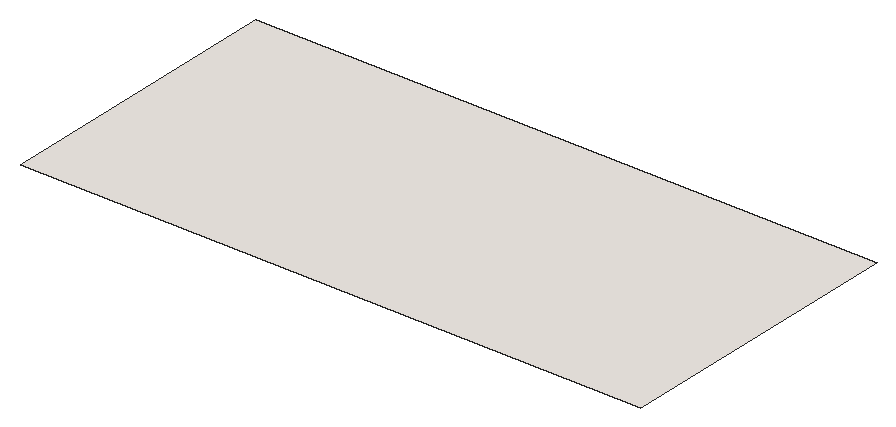
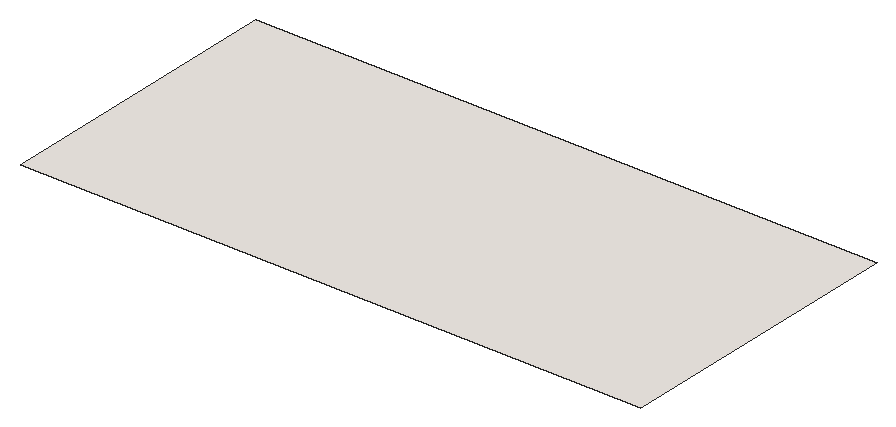
# SketchUp Ruby script. Lengths in inches.
U = 1.inch
M = Sketchup.active_model
def pt(a) = Geom::Point3d.new(a.map { |v| v * U })
def face(e, loops, mat)
  f = e.add_face(loops[0].map { |a| pt(a) })
  loops[1..].each { |l| e.add_face(l.map { |a| pt(a) }).erase! }
  f.material = f.back_material = mat if mat
  f
end
# faces: each face lists its corners as indices into pts; further lists are holes
def faces(e, pts, list, mat = nil) = list.each { |f| face(e, (f[0].is_a?(Array) ? f : [f]).map { |l| l.map { |i| pts[i] } }, mat) }
# xy, xz, yz: faces in a plane at the given z, y or x. An outline is a flat list of corners, or four numbers for a rectangle; further outlines are holes
def ring(l) = l.size == 4 ? [[l[0], l[1]], [l[2], l[1]], [l[2], l[3]], [l[0], l[3]]] : l.each_slice(2).to_a
def flat(e, list, mat, &to3) = list.each { |f| face(e, (f[0].is_a?(Array) ? f : [f]).map { |l| ring(l).map { |u, v| to3.(u, v) } }, mat) }
def xy(e, z, list, mat = nil) = flat(e, list, mat) { |x, y| [x, y, z] }
def xz(e, y, list, mat = nil) = flat(e, list, mat) { |x, z| [x, y, z] }
def yz(e, x, list, mat = nil) = flat(e, list, mat) { |y, z| [x, y, z] }
def lines(e, pts, list) = list.each { |a, b| e.add_line(pt(pts[a]), pt(pts[b])) }
# prism: a flat outline (further loops are holes) pulled along v
def prism(e, loops, v, mat = nil)
  f = face(e, loops, mat); d = Geom::Vector3d.new(v.map { |x| x * U })
  f.pushpull(f.normal.samedirection?(d) ? d.length : -d.length)
end
def box(e, o, s, mat = nil) = prism(e, [[o, [o[0] + s[0], o[1], o[2]], [o[0] + s[0], o[1] + s[1], o[2]], [o[0], o[1] + s[1], o[2]]]], [0, 0, s[2]], mat)
def at(x, y, z, deg = 0) = Geom::Transformation.translation(pt([x, y, z])) * Geom::Transformation.rotation(ORIGIN, Z_AXIS, deg.degrees)
def axes(o, x, y, z) = Geom::Transformation.new([*x, 0, *y, 0, *z, 0, *pt(o).to_a, 1])
def part(name) = M.definitions.add(name)
# library, detail: a bought-in or finely detailed component or shape, given as its bounding box
def library(name, o, s) = part(name).tap { |d| box(d.entities, o, s) }
def detail(e, o, s) = box(e.add_group.entities, o, s)
def put(e, d, t, mat = nil) = e.add_instance(d, t).tap { |i| i.material = mat if mat }
def group(e, t, mat = nil) = e.add_group.tap { |g| g.transformation = t; g.material = mat if mat }.entities
root = M.entities
M.materials.add("0001 AP 9436 AIR BREEZE").color = [243, 237, 232]
xy(root,108,[[23.91,40.5,23.83,40.51,23.75,40.51,23.51,40.54,23.4375,40.55,23.36,40.57,23.28,40.59,23.21,40.61,23.13,40.63,23.06,40.65,22.98,40.68,22.91,40.71,22.84,40.73,22.76,40.77,22.69,40.8,22.625,40.83,22.55,40.87,22.49,40.91,22.35,40.99,22.29,41.04,22.22,41.08,21.98,41.28,21.87,41.39,21.8125,41.45,21.76,41.5,21.61,41.6875,21.5625,41.75,21.52,41.8125,21.48,41.88,21.43,41.95,21.39,42.01,21.36,42.08,21.32,42.15,21.29,42.22,21.25,42.29,21.22,42.37,21.19,42.44,21.17,42.51,21.14,42.59,21.12,42.66,21.0625,42.89,21.05,42.97,21.03,43.05,21.01,43.2,21.01,43.28,21,43.36,21,43.59,21.01,43.67,21.01,43.75,21.04,43.99,21.05,44.0625,21.07,44.14,21.09,44.22,21.11,44.29,21.13,44.37,21.15,44.44,21.18,44.52,21.21,44.59,21.23,44.66,21.27,44.74,21.3,44.81,21.33,44.875,21.37,44.95,21.41,45.01,21.49,45.15,21.54,45.21,21.58,45.28,21.78,45.52,21.89,45.63,21.95,45.6875,22,45.74,22.1875,45.89,22.25,45.9375,22.3125,45.98,22.38,46.02,22.45,46.07,22.51,46.11,22.58,46.14,22.65,46.18,22.72,46.21,22.79,46.25,22.87,46.28,22.94,46.31,23.01,46.33,23.09,46.36,23.16,46.38,23.39,46.4375,23.47,46.45,23.55,46.47,23.7,46.49,23.78,46.49,23.86,46.5,24.09,46.5,24.17,46.49,24.25,46.49,24.49,46.46,24.5625,46.45,24.64,46.43,24.72,46.41,24.79,46.39,24.87,46.37,24.94,46.35,25.02,46.32,25.09,46.29,25.16,46.27,25.24,46.23,25.31,46.2,25.375,46.17,25.45,46.13,25.51,46.09,25.65,46.01,25.71,45.96,25.78,45.92,26.02,45.72,26.13,45.61,26.1875,45.55,26.24,45.5,26.39,45.3125,26.4375,45.25,26.48,45.1875,26.52,45.12,26.57,45.05,26.61,44.99,26.64,44.92,26.68,44.85,26.71,44.78,26.75,44.71,26.78,44.63,26.81,44.56,26.83,44.49,26.86,44.41,26.88,44.34,26.9375,44.11,26.95,44.03,26.97,43.95,26.99,43.8,26.99,43.72,27,43.64,27,43.41,26.99,43.33,26.99,43.25,26.96,43.01,26.95,42.9375,26.93,42.86,26.91,42.78,26.89,42.71,26.87,42.63,26.85,42.56,26.82,42.48,26.79,42.41,26.77,42.34,26.73,42.26,26.7,42.19,26.67,42.125,26.63,42.05,26.59,41.99,26.51,41.85,26.46,41.79,26.42,41.72,26.22,41.48,26.11,41.37,26.05,41.3125,26,41.26,25.8125,41.11,25.75,41.0625,25.6875,41.02,25.62,40.98,25.55,40.93,25.49,40.89,25.42,40.86,25.35,40.82,25.28,40.79,25.21,40.75,25.13,40.72,25.06,40.69,24.99,40.67,24.91,40.64,24.84,40.62,24.61,40.5625,24.53,40.55,24.45,40.53,24.3,40.51,24.22,40.51,24.14,40.5],[68.91,40.5,68.83,40.51,68.75,40.51,68.51,40.54,68.4375,40.55,68.36,40.57,68.28,40.59,68.21,40.61,68.13,40.63,68.06,40.65,67.98,40.68,67.91,40.71,67.84,40.73,67.76,40.77,67.69,40.8,67.625,40.83,67.55,40.87,67.49,40.91,67.35,40.99,67.29,41.04,67.22,41.08,66.98,41.28,66.87,41.39,66.8125,41.45,66.76,41.5,66.61,41.6875,66.5625,41.75,66.52,41.8125,66.48,41.88,66.43,41.95,66.39,42.01,66.36,42.08,66.32,42.15,66.29,42.22,66.25,42.29,66.22,42.37,66.19,42.44,66.17,42.51,66.14,42.59,66.12,42.66,66.0625,42.89,66.05,42.97,66.03,43.05,66.01,43.2,66.01,43.28,66,43.36,66,43.59,66.01,43.67,66.01,43.75,66.04,43.99,66.05,44.0625,66.07,44.14,66.09,44.22,66.11,44.29,66.13,44.37,66.15,44.44,66.18,44.52,66.21,44.59,66.23,44.66,66.27,44.74,66.3,44.81,66.33,44.875,66.37,44.95,66.41,45.01,66.49,45.15,66.54,45.21,66.58,45.28,66.78,45.52,66.89,45.63,66.95,45.6875,67,45.74,67.1875,45.89,67.25,45.9375,67.3125,45.98,67.38,46.02,67.45,46.07,67.51,46.11,67.58,46.14,67.65,46.18,67.72,46.21,67.79,46.25,67.87,46.28,67.94,46.31,68.01,46.33,68.09,46.36,68.16,46.38,68.39,46.4375,68.47,46.45,68.55,46.47,68.7,46.49,68.78,46.49,68.86,46.5,69.09,46.5,69.17,46.49,69.25,46.49,69.49,46.46,69.5625,46.45,69.64,46.43,69.72,46.41,69.79,46.39,69.87,46.37,69.94,46.35,70.02,46.32,70.09,46.29,70.16,46.27,70.24,46.23,70.31,46.2,70.375,46.17,70.45,46.13,70.51,46.09,70.65,46.01,70.71,45.96,70.78,45.92,71.02,45.72,71.13,45.61,71.1875,45.55,71.24,45.5,71.39,45.3125,71.4375,45.25,71.48,45.1875,71.52,45.12,71.57,45.05,71.61,44.99,71.64,44.92,71.68,44.85,71.71,44.78,71.75,44.71,71.78,44.63,71.81,44.56,71.83,44.49,71.86,44.41,71.88,44.34,71.9375,44.11,71.95,44.03,71.97,43.95,71.99,43.8,71.99,43.72,72,43.64,72,43.41,71.99,43.33,71.99,43.25,71.96,43.01,71.95,42.9375,71.93,42.86,71.91,42.78,71.89,42.71,71.87,42.63,71.85,42.56,71.82,42.48,71.79,42.41,71.77,42.34,71.73,42.26,71.7,42.19,71.67,42.125,71.63,42.05,71.59,41.99,71.51,41.85,71.46,41.79,71.42,41.72,71.22,41.48,71.11,41.37,71.05,41.3125,71,41.26,70.8125,41.11,70.75,41.0625,70.6875,41.02,70.62,40.98,70.55,40.93,70.49,40.89,70.42,40.86,70.35,40.82,70.28,40.79,70.21,40.75,70.13,40.72,70.06,40.69,69.99,40.67,69.91,40.64,69.84,40.62,69.61,40.5625,69.53,40.55,69.45,40.53,69.3,40.51,69.22,40.51,69.14,40.5],[113.91,40.5,113.83,40.51,113.75,40.51,113.51,40.54,113.4375,40.55,113.36,40.57,113.28,40.59,113.21,40.61,113.13,40.63,113.06,40.65,112.98,40.68,112.91,40.71,112.84,40.73,112.76,40.77,112.69,40.8,112.625,40.83,112.55,40.87,112.49,40.91,112.35,40.99,112.29,41.04,112.22,41.08,111.98,41.28,111.87,41.39,111.8125,41.45,111.76,41.5,111.61,41.6875,111.5625,41.75,111.52,41.8125,111.48,41.88,111.43,41.95,111.39,42.01,111.36,42.08,111.32,42.15,111.29,42.22,111.25,42.29,111.22,42.37,111.19,42.44,111.17,42.51,111.14,42.59,111.12,42.66,111.0625,42.89,111.05,42.97,111.03,43.05,111.01,43.2,111.01,43.28,111,43.36,111,43.59,111.01,43.67,111.01,43.75,111.04,43.99,111.05,44.0625,111.07,44.14,111.09,44.22,111.11,44.29,111.13,44.37,111.15,44.44,111.18,44.52,111.21,44.59,111.23,44.66,111.27,44.74,111.3,44.81,111.33,44.875,111.37,44.95,111.41,45.01,111.49,45.15,111.54,45.21,111.58,45.28,111.78,45.52,111.89,45.63,111.95,45.6875,112,45.74,112.1875,45.89,112.25,45.9375,112.3125,45.98,112.38,46.02,112.45,46.07,112.51,46.11,112.58,46.14,112.65,46.18,112.72,46.21,112.79,46.25,112.87,46.28,112.94,46.31,113.01,46.33,113.09,46.36,113.16,46.38,113.39,46.4375,113.47,46.45,113.55,46.47,113.7,46.49,113.78,46.49,113.86,46.5,114.09,46.5,114.17,46.49,114.25,46.49,114.49,46.46,114.5625,46.45,114.64,46.43,114.72,46.41,114.79,46.39,114.87,46.37,114.94,46.35,115.02,46.32,115.09,46.29,115.16,46.27,115.24,46.23,115.31,46.2,115.375,46.17,115.45,46.13,115.51,46.09,115.65,46.01,115.71,45.96,115.78,45.92,116.02,45.72,116.13,45.61,116.1875,45.55,116.24,45.5,116.39,45.3125,116.4375,45.25,116.48,45.1875,116.52,45.12,116.57,45.05,116.61,44.99,116.64,44.92,116.68,44.85,116.71,44.78,116.75,44.71,116.78,44.63,116.81,44.56,116.83,44.49,116.86,44.41,116.88,44.34,116.9375,44.11,116.95,44.03,116.97,43.95,116.99,43.8,116.99,43.72,117,43.64,117,43.41,116.99,43.33,116.99,43.25,116.96,43.01,116.95,42.9375,116.93,42.86,116.91,42.78,116.89,42.71,116.87,42.63,116.85,42.56,116.82,42.48,116.79,42.41,116.77,42.34,116.73,42.26,116.7,42.19,116.67,42.125,116.63,42.05,116.59,41.99,116.51,41.85,116.46,41.79,116.42,41.72,116.22,41.48,116.11,41.37,116.05,41.3125,116,41.26,115.8125,41.11,115.75,41.0625,115.6875,41.02,115.62,40.98,115.55,40.93,115.49,40.89,115.42,40.86,115.35,40.82,115.28,40.79,115.21,40.75,115.13,40.72,115.06,40.69,114.99,40.67,114.91,40.64,114.84,40.62,114.61,40.5625,114.53,40.55,114.45,40.53,114.3,40.51,114.22,40.51,114.14,40.5]],"0001 AP 9436 AIR BREEZE")
xy(root,112,[[0,0,183,87]],"0001 AP 9436 AIR BREEZE")
xz(root,40.5,[[113.91,106,113.98,108],[113.98,106,114.0625,108],[114.0625,106,114.14,108]],"0001 AP 9436 AIR BREEZE")
xz(root,40.51,[[113.75,106,113.83,108],[114.22,106,114.3,108]],"0001 AP 9436 AIR BREEZE")
xz(root,46.49,[[113.7,106,113.78,108],[114.17,106,114.25,108]],"0001 AP 9436 AIR BREEZE")
xz(root,46.5,[[113.86,106,113.9375,108],[113.9375,106,114.02,108],[114.02,106,114.09,108]],"0001 AP 9436 AIR BREEZE")
yz(root,111,[[43.36,106,43.4375,108],[43.4375,106,43.52,108],[43.52,106,43.59,108]],"0001 AP 9436 AIR BREEZE")
yz(root,111.01,[[43.2,106,43.28,108],[43.67,106,43.75,108]],"0001 AP 9436 AIR BREEZE")
p = [[113.51,40.54,106],[113.4375,40.55,106],[113.4375,40.55,108],[113.51,40.54,108],[113.59,40.53,106],[113.59,40.53,108],
  [113.67,40.52,106],[113.67,40.52,108],[113.75,40.51,106],[113.75,40.51,108],[113.91,40.5,106],[113.83,40.51,106],
  [113.83,40.51,108],[113.91,40.5,108],[114.22,40.51,106],[114.14,40.5,106],[114.14,40.5,108],[114.22,40.51,108],
  [114.375,40.52,106],[114.3,40.51,106],[114.3,40.51,108],[114.375,40.52,108],[114.45,40.53,106],[114.45,40.53,108],
  [114.53,40.55,106],[114.53,40.55,108],[114.61,40.5625,106],[114.61,40.5625,108],[113.13,40.63,106],[113.06,40.65,106],
  [113.06,40.65,108],[113.13,40.63,108],[113.21,40.61,106],[113.21,40.61,108],[113.28,40.59,106],[113.28,40.59,108],
  [113.36,40.57,106],[113.36,40.57,108],[114.68,40.58,106],[114.68,40.58,108],[114.76,40.6,106],[114.76,40.6,108],
  [114.84,40.62,106],[114.84,40.62,108],[114.91,40.64,106],[114.91,40.64,108],[114.99,40.67,106],[114.99,40.67,108],
  [112.84,40.73,106],[112.76,40.77,106],[112.76,40.77,108],[112.84,40.73,108],[112.91,40.71,106],[112.91,40.71,108],
  [112.98,40.68,106],[112.98,40.68,108],[115.06,40.69,106],[115.06,40.69,108],[115.13,40.72,106],[115.13,40.72,108],
  [115.21,40.75,106],[115.21,40.75,108],[112.625,40.83,106],[112.55,40.87,106],[112.55,40.87,108],[112.625,40.83,108],
  [112.69,40.8,106],[112.69,40.8,108],[115.28,40.79,106],[115.28,40.79,108],[115.35,40.82,106],[115.35,40.82,108],
  [115.42,40.86,106],[115.42,40.86,108],[112.49,40.91,106],[112.42,40.95,106],[112.42,40.95,108],[112.49,40.91,108],
  [115.49,40.89,106],[115.49,40.89,108],[115.55,40.93,106],[115.55,40.93,108],[115.62,40.98,106],[115.62,40.98,108],
  [112.29,41.04,106],[112.22,41.08,106],[112.22,41.08,108],[112.29,41.04,108],[112.35,40.99,106],[112.35,40.99,108],
  [115.6875,41.02,106],[115.6875,41.02,108],[115.75,41.0625,106],[115.75,41.0625,108],[112.16,41.13,106],[112.1,41.18,106],
  [112.1,41.18,108],[112.16,41.13,108],[115.8125,41.11,106],[115.8125,41.11,108],[115.875,41.16,106],[115.875,41.16,108],
  [112.04,41.23,106],[111.98,41.28,106],[111.98,41.28,108],[112.04,41.23,108],[115.9375,41.21,106],[115.9375,41.21,108],
  [116,41.26,106],[116,41.26,108],[111.92,41.34,106],[111.87,41.39,106],[111.87,41.39,108],[111.92,41.34,108],
  [116.05,41.3125,106],[116.05,41.3125,108],[116.11,41.37,106],[116.11,41.37,108],[111.8125,41.45,106],[111.76,41.5,106],
  [111.76,41.5,108],[111.8125,41.45,108],[116.16,41.42,106],[116.16,41.42,108],[116.22,41.48,106],[116.22,41.48,108],
  [111.71,41.5625,106],[111.71,41.5625,108],[116.27,41.54,106],[116.27,41.54,108],[116.32,41.6,106],[116.32,41.6,108],
  [111.66,41.625,106],[111.61,41.6875,106],[111.61,41.6875,108],[111.66,41.625,108],[116.37,41.66,106],[116.37,41.66,108],
  [111.5625,41.75,106],[111.52,41.8125,106],[111.52,41.8125,108],[111.5625,41.75,108],[116.42,41.72,106],[116.42,41.72,108],
  [116.46,41.79,106],[116.46,41.79,108],[111.48,41.88,106],[111.48,41.88,108],[116.51,41.85,106],[116.51,41.85,108],
  [111.43,41.95,106],[111.39,42.01,106],[111.39,42.01,108],[111.43,41.95,108],[116.55,41.92,106],[116.55,41.92,108],
  [116.59,41.99,106],[116.59,41.99,108],[111.36,42.08,106],[111.36,42.08,108],[116.63,42.05,106],[116.63,42.05,108],
  [111.32,42.15,106],[111.32,42.15,108],[116.67,42.125,106],[116.67,42.125,108],[116.7,42.19,106],[116.7,42.19,108],
  [111.29,42.22,106],[111.25,42.29,106],[111.25,42.29,108],[111.29,42.22,108],[116.73,42.26,106],[116.73,42.26,108],
  [111.22,42.37,106],[111.22,42.37,108],[116.77,42.34,106],[116.77,42.34,108],[116.79,42.41,106],[116.79,42.41,108],
  [111.19,42.44,106],[111.17,42.51,106],[111.17,42.51,108],[111.19,42.44,108],[116.82,42.48,106],[116.82,42.48,108],
  [111.14,42.59,106],[111.14,42.59,108],[116.85,42.56,106],[116.85,42.56,108],[111.12,42.66,106],[111.12,42.66,108],
  [116.87,42.63,106],[116.87,42.63,108],[116.89,42.71,106],[116.89,42.71,108],[111.1,42.74,106],[111.08,42.82,106],
  [111.08,42.82,108],[111.1,42.74,108],[116.91,42.78,106],[116.91,42.78,108],[111.0625,42.89,106],[111.0625,42.89,108],
  [116.93,42.86,106],[116.93,42.86,108],[111.05,42.97,106],[111.05,42.97,108],[116.95,42.9375,106],[116.95,42.9375,108],
  [116.96,43.01,106],[116.96,43.01,108],[111.03,43.05,106],[111.02,43.125,106],[111.02,43.125,108],[111.03,43.05,108],
  [116.97,43.09,106],[116.97,43.09,108],[111.01,43.2,106],[111.01,43.2,108],[116.98,43.17,106],[116.98,43.17,108],
  [116.99,43.25,106],[116.99,43.25,108],[111.01,43.28,106],[111,43.36,106],[111,43.36,108],[111.01,43.28,108],
  [111,43.59,106],[111.01,43.67,106],[111.01,43.67,108],[111,43.59,108],[111.01,43.75,106],[111.02,43.83,106],
  [111.02,43.83,108],[111.01,43.75,108],[111.03,43.91,106],[111.03,43.91,108],[116.98,43.875,106],[116.99,43.8,106],
  [116.99,43.8,108],[116.98,43.875,108],[111.04,43.99,106],[111.04,43.99,108],[116.97,43.95,106],[116.97,43.95,108],
  [111.05,44.0625,106],[111.05,44.0625,108],[116.9375,44.11,106],[116.95,44.03,106],[116.95,44.03,108],[116.9375,44.11,108],
  [111.07,44.14,106],[111.07,44.14,108],[111.09,44.22,106],[111.09,44.22,108],[116.92,44.18,106],[116.92,44.18,108],
  [111.11,44.29,106],[111.11,44.29,108],[116.9,44.26,106],[116.9,44.26,108],[111.13,44.37,106],[111.13,44.37,108],
  [116.86,44.41,106],[116.88,44.34,106],[116.88,44.34,108],[116.86,44.41,108],[111.15,44.44,106],[111.15,44.44,108],
  [111.18,44.52,106],[111.18,44.52,108],[116.83,44.49,106],[116.83,44.49,108],[111.21,44.59,106],[111.21,44.59,108],
  [116.81,44.56,106],[116.81,44.56,108],[111.23,44.66,106],[111.23,44.66,108],[116.75,44.71,106],[116.78,44.63,106],
  [116.78,44.63,108],[116.75,44.71,108],[111.27,44.74,106],[111.27,44.74,108],[111.3,44.81,106],[111.3,44.81,108],
  [116.71,44.78,106],[116.71,44.78,108],[111.33,44.875,106],[111.33,44.875,108],[116.64,44.92,106],[116.68,44.85,106],
  [116.68,44.85,108],[116.64,44.92,108],[111.37,44.95,106],[111.37,44.95,108],[111.41,45.01,106],[111.41,45.01,108],
  [116.61,44.99,106],[116.61,44.99,108],[111.45,45.08,106],[111.45,45.08,108],[116.57,45.05,106],[116.57,45.05,108],
  [111.49,45.15,106],[111.49,45.15,108],[111.54,45.21,106],[111.54,45.21,108],[116.48,45.1875,106],[116.52,45.12,106],
  [116.52,45.12,108],[116.48,45.1875,108],[111.58,45.28,106],[111.58,45.28,108],[116.4375,45.25,106],[116.4375,45.25,108],
  [111.63,45.34,106],[111.63,45.34,108],[111.68,45.4,106],[111.68,45.4,108],[116.34,45.375,106],[116.39,45.3125,106],
  [116.39,45.3125,108],[116.34,45.375,108],[111.73,45.46,106],[111.73,45.46,108],[116.24,45.5,106],[116.29,45.4375,106],
  [116.29,45.4375,108],[116.24,45.5,108],[111.78,45.52,106],[111.78,45.52,108],[111.84,45.58,106],[111.84,45.58,108],
  [116.1875,45.55,106],[116.1875,45.55,108],[111.89,45.63,106],[111.89,45.63,108],[111.95,45.6875,106],[111.95,45.6875,108],
  [116.08,45.66,106],[116.13,45.61,106],[116.13,45.61,108],[116.08,45.66,108],[112,45.74,106],[112,45.74,108],
  [112.0625,45.79,106],[112.0625,45.79,108],[115.96,45.77,106],[116.02,45.72,106],[116.02,45.72,108],[115.96,45.77,108],
  [112.125,45.84,106],[112.125,45.84,108],[112.1875,45.89,106],[112.1875,45.89,108],[115.84,45.87,106],[115.9,45.82,106],
  [115.9,45.82,108],[115.84,45.87,108],[70.71,45.96,106],[70.78,45.92,106],[70.78,45.92,108],[70.71,45.96,108],
  [112.25,45.9375,106],[112.25,45.9375,108],[112.3125,45.98,106],[112.3125,45.98,108],[115.71,45.96,106],[115.78,45.92,106],
  [115.78,45.92,108],[115.71,45.96,108],[70.51,46.09,106],[70.58,46.05,106],[70.58,46.05,108],[70.51,46.09,108],
  [70.65,46.01,106],[70.65,46.01,108],[112.38,46.02,106],[112.38,46.02,108],[112.45,46.07,106],[112.45,46.07,108],
  [115.51,46.09,106],[115.58,46.05,106],[115.58,46.05,108],[115.51,46.09,108],[115.65,46.01,106],[115.65,46.01,108],
  [70.375,46.17,106],[70.45,46.13,106],[70.45,46.13,108],[70.375,46.17,108],[112.51,46.11,106],[112.51,46.11,108],
  [112.58,46.14,106],[112.58,46.14,108],[112.65,46.18,106],[112.65,46.18,108],[115.375,46.17,106],[115.45,46.13,106],
  [115.45,46.13,108],[115.375,46.17,108],[70.16,46.27,106],[70.24,46.23,106],[70.24,46.23,108],[70.16,46.27,108],
  [70.31,46.2,106],[70.31,46.2,108],[112.72,46.21,106],[112.72,46.21,108],[112.79,46.25,106],[112.79,46.25,108],
  [112.87,46.28,106],[112.87,46.28,108],[115.16,46.27,106],[115.24,46.23,106],[115.24,46.23,108],[115.16,46.27,108],
  [115.31,46.2,106],[115.31,46.2,108],[70.02,46.32,106],[70.09,46.29,106],[70.09,46.29,108],[70.02,46.32,108],
  [112.94,46.31,106],[112.94,46.31,108],[113.01,46.33,106],[113.01,46.33,108],[113.09,46.36,106],[113.09,46.36,108],
  [114.87,46.37,106],[114.94,46.35,106],[114.94,46.35,108],[114.87,46.37,108],[115.02,46.32,106],[115.02,46.32,108],
  [115.09,46.29,106],[115.09,46.29,108],[113.16,46.38,106],[113.16,46.38,108],[113.24,46.4,106],[113.24,46.4,108],
  [113.32,46.42,106],[113.32,46.42,108],[113.39,46.4375,106],[113.39,46.4375,108],[113.47,46.45,106],[113.47,46.45,108],
  [114.49,46.46,106],[114.5625,46.45,106],[114.5625,46.45,108],[114.49,46.46,108],[114.64,46.43,106],[114.64,46.43,108],
  [114.72,46.41,106],[114.72,46.41,108],[114.79,46.39,106],[114.79,46.39,108],[113.55,46.47,106],[113.55,46.47,108],
  [113.625,46.48,106],[113.625,46.48,108],[113.7,46.49,106],[113.7,46.49,108],[113.78,46.49,106],[113.86,46.5,106],
  [113.86,46.5,108],[113.78,46.49,108],[114.09,46.5,106],[114.17,46.49,106],[114.17,46.49,108],[114.09,46.5,108],
  [114.25,46.49,106],[114.33,46.48,106],[114.33,46.48,108],[114.25,46.49,108],[114.41,46.47,106],[114.41,46.47,108]]
faces(root,p,[[0,1,2,3],[4,0,3,5],[6,4,5,7],[8,6,7,9],[10,11,12,13],[14,15,16,17],[18,19,20,21],[22,18,21,23],
  [24,22,23,25],[26,24,25,27],[28,29,30,31],[32,28,31,33],[34,32,33,35],[36,34,35,37],[1,36,37,2],[38,26,27,39],
  [40,38,39,41],[42,40,41,43],[44,42,43,45],[46,44,45,47],[48,49,50,51],[52,48,51,53],[54,52,53,55],[29,54,55,30],
  [56,46,47,57],[58,56,57,59],[60,58,59,61],[62,63,64,65],[66,62,65,67],[49,66,67,50],[68,60,61,69],[70,68,69,71],
  [72,70,71,73],[74,75,76,77],[63,74,77,64],[78,72,73,79],[80,78,79,81],[82,80,81,83],[84,85,86,87],[88,84,87,89],
  [75,88,89,76],[90,82,83,91],[92,90,91,93],[94,95,96,97],[85,94,97,86],[98,92,93,99],[100,98,99,101],[102,103,104,105],
  [95,102,105,96],[106,100,101,107],[108,106,107,109],[110,111,112,113],[103,110,113,104],[114,108,109,115],[116,114,115,117],[118,119,120,121],
  [111,118,121,112],[122,116,117,123],[124,122,123,125],[119,126,127,120],[128,124,125,129],[130,128,129,131],[132,133,134,135],[126,132,135,127],
  [136,130,131,137],[138,139,140,141],[133,138,141,134],[142,136,137,143],[144,142,143,145],[139,146,147,140],[148,144,145,149],[150,151,152,153],
  [146,150,153,147],[154,148,149,155],[156,154,155,157],[151,158,159,152],[160,156,157,161],[158,162,163,159],[164,160,161,165],[166,164,165,167],
  [168,169,170,171],[162,168,171,163],[172,166,167,173],[169,174,175,170],[176,172,173,177],[178,176,177,179],[180,181,182,183],[174,180,183,175],
  [184,178,179,185],[181,186,187,182],[188,184,185,189],[186,190,191,187],[192,188,189,193],[194,192,193,195],[196,197,198,199],[190,196,199,191],
  [200,194,195,201],[197,202,203,198],[204,200,201,205],[202,206,207,203],[208,204,205,209],[210,208,209,211],[212,213,214,215],[206,212,215,207],
  [216,210,211,217],[213,218,219,214],[220,216,217,221],[222,220,221,223],[224,225,226,227],[228,229,230,231],[232,233,234,235],[233,236,237,234],
  [238,239,240,241],[236,242,243,237],[244,238,241,245],[242,246,247,243],[248,249,250,251],[249,244,245,250],[246,252,253,247],[252,254,255,253],
  [256,248,251,257],[254,258,259,255],[260,256,257,261],[258,262,263,259],[264,265,266,267],[265,260,261,266],[262,268,269,263],[268,270,271,269],
  [272,264,267,273],[270,274,275,271],[276,272,273,277],[274,278,279,275],[280,281,282,283],[281,276,277,282],[278,284,285,279],[284,286,287,285],
  [288,280,283,289],[286,290,291,287],[292,293,294,295],[293,288,289,294],[290,296,297,291],[296,298,299,297],[300,292,295,301],[298,302,303,299],
  [304,300,301,305],[302,306,307,303],[306,308,309,307],[310,311,312,313],[311,304,305,312],[308,314,315,309],[316,310,313,317],[314,318,319,315],
  [318,320,321,319],[322,323,324,325],[323,316,317,324],[320,326,327,321],[328,329,330,331],[329,322,325,330],[326,332,333,327],[332,334,335,333],
  [336,328,331,337],[334,338,339,335],[338,340,341,339],[342,343,344,345],[343,336,337,344],[340,346,347,341],[346,348,349,347],[350,351,352,353],
  [351,342,345,352],[348,354,355,349],[354,356,357,355],[358,359,360,361],[359,350,353,360],[362,363,364,365],[356,366,367,357],[366,368,369,367],
  [370,371,372,373],[371,358,361,372],[374,375,376,377],[375,378,379,376],[378,362,365,379],[368,380,381,369],[380,382,383,381],[384,385,386,387],
  [385,388,389,386],[388,370,373,389],[390,391,392,393],[391,374,377,392],[382,394,395,383],[394,396,397,395],[396,398,399,397],[400,401,402,403],
  [401,384,387,402],[404,405,406,407],[405,408,409,406],[408,390,393,409],[398,410,411,399],[410,412,413,411],[412,414,415,413],[416,417,418,419],
  [417,420,421,418],[420,400,403,421],[422,423,424,425],[423,404,407,424],[414,426,427,415],[426,428,429,427],[428,430,431,429],[432,433,434,435],
  [433,436,437,434],[436,438,439,437],[438,416,419,439],[430,440,441,431],[440,442,443,441],[442,444,445,443],[444,446,447,445],[446,448,449,447],
  [450,451,452,453],[451,454,455,452],[454,456,457,455],[456,458,459,457],[458,432,435,459],[448,460,461,449],[460,462,463,461],[462,464,465,463],
  [466,467,468,469],[470,471,472,473],[474,475,476,477],[475,478,479,476],[478,450,453,479]],"0001 AP 9436 AIR BREEZE")
